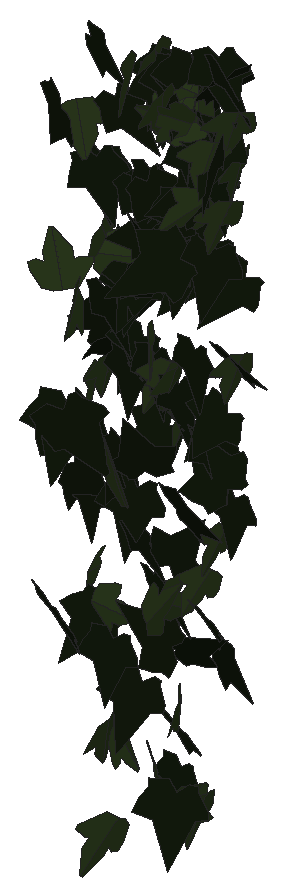
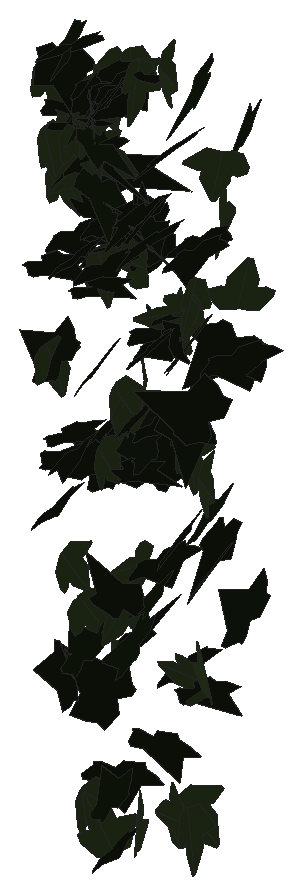
# SketchUp Ruby script. Lengths in inches.
U = 1.inch
M = Sketchup.active_model
def pt(a) = Geom::Point3d.new(a.map { |v| v * U })
def face(e, loops, mat)
  f = e.add_face(loops[0].map { |a| pt(a) })
  loops[1..].each { |l| e.add_face(l.map { |a| pt(a) }).erase! }
  f.material = f.back_material = mat if mat
  f
end
# faces: each face lists its corners as indices into pts; further lists are holes
def faces(e, pts, list, mat = nil) = list.each { |f| face(e, (f[0].is_a?(Array) ? f : [f]).map { |l| l.map { |i| pts[i] } }, mat) }
# xy, xz, yz: faces in a plane at the given z, y or x. An outline is a flat list of corners, or four numbers for a rectangle; further outlines are holes
def ring(l) = l.size == 4 ? [[l[0], l[1]], [l[2], l[1]], [l[2], l[3]], [l[0], l[3]]] : l.each_slice(2).to_a
def flat(e, list, mat, &to3) = list.each { |f| face(e, (f[0].is_a?(Array) ? f : [f]).map { |l| ring(l).map { |u, v| to3.(u, v) } }, mat) }
def xy(e, z, list, mat = nil) = flat(e, list, mat) { |x, y| [x, y, z] }
def xz(e, y, list, mat = nil) = flat(e, list, mat) { |x, z| [x, y, z] }
def yz(e, x, list, mat = nil) = flat(e, list, mat) { |y, z| [x, y, z] }
def lines(e, pts, list) = list.each { |a, b| e.add_line(pt(pts[a]), pt(pts[b])) }
# prism: a flat outline (further loops are holes) pulled along v
def prism(e, loops, v, mat = nil)
  f = face(e, loops, mat); d = Geom::Vector3d.new(v.map { |x| x * U })
  f.pushpull(f.normal.samedirection?(d) ? d.length : -d.length)
end
def box(e, o, s, mat = nil) = prism(e, [[o, [o[0] + s[0], o[1], o[2]], [o[0] + s[0], o[1] + s[1], o[2]], [o[0], o[1] + s[1], o[2]]]], [0, 0, s[2]], mat)
def at(x, y, z, deg = 0) = Geom::Transformation.translation(pt([x, y, z])) * Geom::Transformation.rotation(ORIGIN, Z_AXIS, deg.degrees)
def axes(o, x, y, z) = Geom::Transformation.new([*x, 0, *y, 0, *z, 0, *pt(o).to_a, 1])
def part(name) = M.definitions.add(name)
# library, detail: a bought-in or finely detailed component or shape, given as its bounding box
def library(name, o, s) = part(name).tap { |d| box(d.entities, o, s) }
def detail(e, o, s) = box(e.add_group.entities, o, s)
def put(e, d, t, mat = nil) = e.add_instance(d, t).tap { |i| i.material = mat if mat }
def group(e, t, mat = nil) = e.add_group.tap { |g| g.transformation = t; g.material = mat if mat }.entities
root = M.entities
M.materials.add("efeu1").color = [18, 25, 13]
M.materials.add("efeu2").color = [43, 57, 29]
c1 = part("ivyleaf_10")
p = [[0,0.5,-0.03],[-0.0625,2.02,-0.43],[-0.19,2.01,-0.46],[-0.54,1.05,-0.29],[-0.52,0.625,-0.18],[-0.83,0.76,-0.28],
  [-1.16,0.64,-0.33],[-1.15,0.33,-0.24],[-0.77,-0.39,0.02],[-0.3,-0.51,0.16],[0.04,-0.48,0.23],[-0.02,2.01,-0.4375],
  [-0.06,2.01,-0.43],[0.04,-0.49,0.23],[0.67,-0.49,0.14],[1.38,0.36,-0.2],[1.375,0.51,-0.24],[0.81,0.65,-0.19],
  [0.62,0.59,-0.15],[0.6,1.09,-0.28],[0.5,1.23,-0.31]]
faces(c1.entities,p,[[0,1,2,3,4,5,6,7,8,9,10],[11,12,0,13,14,15,16,17,18,19,20]],"efeu2")
c2 = part("ivyleaf_9")
p = [[1.54,2.16,1.25],[1.36,2.04,1.19],[-0.21,0.99,0.68],[-0.71,1.11,0.82],[-0.85,0.86,0.67],[-0.8,0.17,0.21],
  [-0.9,-0.01,0.1],[-0.67,-0.16,-0.02],[-0.08,-0.08,-0.05],[-0.03,-0.6,-0.4],[0.65,-0.88,-0.66],[0.83,-0.6,-0.49],
  [1.29,-0.42,-0.43],[1.8125,-0.07,-0.26],[1.21,0.44,0.15]]
faces(c2.entities,p,[[0,1,2,3,4,5,6,7,8,9,10,11,12,13,14]],"efeu1")
put(root,c1,axes([528.05,122.93,226.38],[-0.82158,0.69084,-0.51551],[-0.39036,0.33675,1.07342],[0.76852,0.90958,-0.00587]))
put(root,c1,axes([524.125,124.99,233.47],[-0.13432,0.38401,-1.0691],[0.2143,-1.04865,-0.40359],[-1.11557,-0.24768,0.05119]))
put(root,c2,axes([523.31,125.25,227.76],[-0.44076,-1.03489,-0.11415],[0.04301,0.10575,-1.12484],[1.04028,-0.44285,-0.00185]))
put(root,c2,axes([523.81,124.54,228.03],[-0.22106,-0.48104,-1.08794],[0.56667,0.93036,-0.5265],[1.0459,-0.60574,0.05532]))
put(root,c2,axes([521.58,126.45,217.07],[0.38586,-0.75336,0.79815],[0.49333,-0.63671,-0.83948],[0.98042,0.61688,0.10828]))
put(root,c1,axes([524.64,126.52,207.5],[-0.23778,-0.90858,0.68289],[-0.07381,-0.68385,-0.93556],[1.13419,-0.23498,0.08228]))
put(root,c2,axes([527.59,127.25,235.54],[-0.92071,-0.44136,0.53496],[-0.48506,-0.22567,-1.02101],[0.49568,-1.04065,-0.00548]))
put(root,c2,axes([520.4,128.47,239.76],[0.04113,-0.61141,0.89089],[0.11295,-0.88422,-0.61205],[1.07459,0.11634,0.03024]))
put(root,c2,axes([526.9,128.12,209.15],[-0.64224,-0.76315,-0.42743],[0.2906,0.314,-0.99726],[0.82502,-0.70468,0.01853]))
put(root,c2,axes([527,128.16,222.95],[0.48538,-0.48585,0.89186],[0.66554,-0.5945,-0.68607],[0.76716,0.82315,0.03091]))
put(root,c2,axes([523.32,128.32,215.22],[-0.15697,-0.9643,0.02792],[-0.00409,-0.02762,-0.97699],[0.9647,-0.15702,0.0004]))
put(root,c1,axes([527.36,127.64,213.96],[0.4042,-0.81495,-0.41775],[-0.07641,0.42502,-0.90308],[0.91259,0.39654,0.10941]))
put(root,c1,axes([520.98,127.72,232.23],[0.76284,0.74931,0.11152],[-0.08398,-0.07364,1.06928],[0.7529,-0.76742,0.00628]))
put(root,c1,axes([526.41,127.1,218.1],[0.03617,0.22167,-0.982],[0.18316,0.96479,0.22453],[0.98991,-0.18661,-0.00566]))
put(root,c2,axes([525.27,127.54,233.92],[0.06716,0.70227,-0.87889],[-0.07759,0.88125,0.69822],[1.12232,0.0189,0.10086]))
put(root,c1,axes([527.23,129.23,237.1875],[-0.20712,-0.47742,0.89381],[-0.34689,-0.82377,-0.52039],[0.9521,-0.40399,0.00484]))
put(root,c2,axes([525.67,129.17,215.49],[-0.16332,-1.08391,-0.06907],[0.01401,-0.07194,1.09587],[-1.08602,0.16207,0.02452]))
put(root,c1,axes([526.28,129.19,240.88],[-0.45119,-0.04257,-0.89484],[-0.78436,-0.4653,0.41762],[-0.43282,0.88759,0.17601]))
put(root,c2,axes([524.46,129.01,223.66],[0.66107,0.19822,0.71645],[-0.72383,-0.04672,0.6808],[0.16931,-0.97372,0.11318]))
put(root,c1,axes([525.6,128.76,241.8125],[0.01224,-0.98949,-0.23253],[0.04073,0.23284,-0.98866],[1.01563,0.00259,0.04245]))
put(root,c1,axes([523.38,129.43,242.38],[0.36501,-0.60969,0.76872],[0.47856,-0.60538,-0.70737],[0.85653,0.59806,0.06763]))
put(root,c2,axes([524.375,129.59,233.91],[-0.36953,-0.23006,0.96265],[0.47782,-0.94135,-0.04155],[0.86678,0.42084,0.43331]))
put(root,c1,axes([527.19,129.4375,208.32],[0.05239,-1.06977,0.20179],[0.0094,-0.20157,-1.07105],[1.08859,0.05322,-0.00046]))
put(root,c2,axes([521.48,129.8125,215.42],[-0.75245,-0.58306,0.12384],[-0.09953,-0.07374,-0.95191],[0.5877,-0.759,-0.00265]))
put(root,c1,axes([527.54,129.65,239.68],[-0.56199,-0.75208,0.30846],[-0.03648,-0.35129,-0.92297],[0.81206,-0.53626,0.17201]))
put(root,c1,axes([520.67,129.3,239.35],[0.73743,0.69098,0.18934],[0.1294,0.13879,-1.01049],[-0.70467,0.74859,0.01258]))
put(root,c2,axes([526.95,129.5625,237.52],[-0.94111,0.29635,0.29843],[-0.28157,0.09938,-0.98662],[-0.31242,-0.98228,-0.00978]))
put(root,c2,axes([520.66,129.97,221.14],[0.21557,-0.86108,0.23473],[0.02361,-0.23589,-0.88703],[0.89218,0.2143,-0.03324]))
put(root,c2,axes([525.78,130.06,233.94],[-0.22906,-0.94928,0.0558],[0.0273,-0.06394,-0.97565],[0.95053,-0.22693,0.04147]))
put(root,c2,axes([521.81,129.75,230.93],[0.5139,-0.90185,-0.06053],[-0.02558,0.0551,-1.03798],[0.90352,0.51451,0.00505]))
put(root,c2,axes([523.51,129.92,212.54],[-0.86262,-0.51536,-0.33613],[0.28798,0.17335,-1.00485],[0.54373,-0.90942,-0.00106]))
put(root,c2,axes([527.5,129.93,239.87],[-0.6685,0.03235,-0.80034],[0.79361,-0.11444,-0.66751],[-0.10848,-1.03651,0.04872]))
put(root,c1,axes([524.52,129.68,233.44],[0.06923,-0.03854,1.09488],[1.09536,0.02307,-0.06845],[-0.0206,1.09682,0.03991]))
put(root,c1,axes([525.54,129,217.65],[-0.15498,-0.64223,-0.88155],[0.24334,0.8476,-0.66028],[1.06319,-0.28762,0.02262]))
put(root,c1,axes([521.6,129.79,215.79],[-0.06161,-0.14923,-0.94753],[0.91503,-0.29398,-0.0132],[-0.28775,-0.90288,0.16091]))
put(root,c2,axes([522.63,130.26,227.44],[0.11146,-0.86515,0.39633],[0.08959,-0.38773,-0.87156],[0.94738,0.13845,0.03579]))
put(root,c2,axes([520.71,129.15,222.49],[0.27625,-0.36518,-0.96289],[-0.57807,0.77007,-0.4579],[0.85227,0.64068,0.00153]))
put(root,c2,axes([525.0625,130.19,235.4],[-0.62155,-0.40287,-0.62601],[0.66837,0.05712,-0.70038],[0.32782,-0.88031,0.24104]))
put(root,c1,axes([525.47,129.42,240.3125],[0.99684,0.20328,-0.47278],[0.40809,0.31566,0.99617],[0.31354,-1.05715,0.20654]))
put(root,c1,axes([527.91,130.18,236.74],[-0.22239,-0.9539,0.34583],[-0.03989,-0.34555,-0.97876],[1.01387,-0.22283,0.03735]))
put(root,c2,axes([521.3,129.58,242.93],[0.78232,-0.42719,-0.51522],[-0.41356,0.31458,-0.8888],[0.52621,0.88233,0.06745]))
put(root,c2,axes([524.18,129.78,234.72],[-0.74461,0.53945,0.32451],[-0.31965,0.10905,-0.91471],[-0.54234,-0.8049,0.09357]))
put(root,c1,axes([522.03,130.21,209.45],[0.24571,-0.08568,1.02242],[1.00044,-0.21322,-0.2583],[0.22761,1.02969,0.03159]))
put(root,c2,axes([527.11,130.45,234.33],[-0.34737,-0.96548,-0.06332],[0.01068,0.06345,-1.026],[0.96749,-0.34734,-0.01141]))
put(root,c1,axes([526.03,130.28,241.25],[-0.70517,-0.59037,0.36839],[-0.149,-0.38422,-0.90094],[0.67974,-0.69668,0.18469]))
put(root,c2,axes([527.4375,130.51,240.04],[-0.67206,-0.71263,-0.16812],[0.15229,0.08717,-0.97825],[0.71618,-0.68726,0.05026]))
put(root,c1,axes([523.59,130.53,228.95],[-0.30792,0.42784,-0.84012],[0.33795,-0.77497,-0.51853],[-0.88013,-0.44725,0.09482]))
put(root,c1,axes([525.66,130.1,207.25],[-0.77015,-0.42954,0.52529],[0.51386,0.14972,0.87584],[-0.44314,0.92013,0.1027]))
put(root,c2,axes([524.43,130.48,241.76],[-0.20291,-0.97376,-0.16203],[0.02509,0.16028,-0.99465],[0.98683,-0.2043,-0.00803]))
put(root,c1,axes([524.94,130.29,227.68],[0.108,-0.95409,0.09059],[0.01397,-0.08959,-0.96018],[0.95828,0.10883,0.00378]))
put(root,c1,axes([528.32,130.29,241.16],[-0.47391,-0.85715,0.19311],[-0.10186,-0.16433,-0.97939],[0.87271,-0.48464,-0.00945]))
put(root,c2,axes([522.7,130.69,221.24],[-0.30401,-1.01642,-0.05268],[0.01513,0.05047,-1.06091],[1.01767,-0.30439,0.00003]))
put(root,c1,axes([523.87,130.52,208.03],[-0.58296,0.44962,0.68947],[0.55492,-0.40933,0.73613],[0.60794,0.80477,-0.01078]))
put(root,c2,axes([522.93,130.25,219.67],[0.61871,-0.66751,-0.06586],[-0.01633,0.07458,-0.90933],[0.67055,0.61772,0.03862]))
put(root,c1,axes([524.24,130.68,227.51],[-0.24512,-0.73679,0.54659],[0.02961,-0.57182,-0.75753],[0.91692,-0.1785,0.17058]))
put(root,c2,axes([520.11,130.88,223.9],[0.07427,-0.79347,0.61327],[0.17046,-0.59601,-0.79178],[0.98825,0.16243,0.09049]))
put(root,c2,axes([527.8,130.26,223.42],[-0.85081,-0.62406,-0.02234],[-0.00632,-0.02913,1.05495],[-0.62442,0.8506,0.01975]))
put(root,c2,axes([524.23,130.82,224.82],[-0.77445,-0.42705,0.3107],[-0.23226,-0.21986,-0.88113],[0.4743,-0.80496,0.07584]))
put(root,c1,axes([521.46,130.24,209.65],[0.09529,-1.02806,-0.19432],[-0.02142,0.19317,-1.03247],[1.04605,0.09761,-0.00344]))
put(root,c2,axes([525.75,130.8,228.875],[0.22779,-0.91816,0.22903],[0.02551,-0.22953,-0.94553],[0.94595,0.22729,-0.02966]))
put(root,c2,axes([521.65,131.11,222.34],[-0.03199,-0.80115,0.61232],[-0.02216,-0.61192,-0.80178],[1.00811,-0.03887,0.00181]))
put(root,c1,axes([525.78,130.48,233.55],[-0.10448,-0.95509,0.05949],[-0.00492,-0.05931,-0.96079],[0.95693,-0.10458,0.00156]))
put(root,c2,axes([522.03,130.28,240],[0.49496,-0.78164,-0.39133],[0.05385,0.47612,-0.88289],[0.87247,0.41404,0.2765]))
put(root,c1,axes([520.22,130.84,216.39],[0.18752,-0.56593,-0.73593],[0.42453,-0.61542,0.58143],[-0.82561,-0.44498,0.13182]))
put(root,c2,axes([522.86,130.9375,231.7],[-0.49023,-0.83607,0.06848],[-0.01952,-0.06793,-0.96904],[0.83865,-0.49031,0.01748]))
put(root,c2,axes([524.875,130.875,242.01],[-0.33972,-0.94987,-0.04401],[0.01231,0.04234,-1.00879],[0.95081,-0.33994,-0.00267]))
put(root,c1,axes([521.38,130.09,233.51],[0.0962,-0.84611,-0.48465],[0.13742,0.49391,-0.835],[0.96536,0.01401,0.16716]))
put(root,c2,axes([525.125,130.83,235.82],[-0.18444,-0.95277,-0.0685],[0.01328,0.0672,-0.97045],[0.95513,-0.18492,0.00027]))
put(root,c2,axes([524.42,130.95,242.09],[-0.50013,-0.85702,0.03239],[-0.01383,-0.02943,-0.99227],[0.85752,-0.50032,0.00289]))
put(root,c2,axes([523.75,130.28,236.51],[0.40042,-0.75278,-0.57248],[-0.06336,0.59893,-0.83188],[0.94361,0.35966,0.18707]))
put(root,c1,axes([520.18,131,225.7],[0.35334,-0.64675,0.74932],[0.50447,-0.56689,-0.72717],[0.85164,0.60413,0.11985]))
put(root,c2,axes([526.26,130.79,236.04],[-0.96258,-0.14515,0.08264],[-0.08254,-0.00689,-0.97345],[0.14521,-0.9661,-0.00547]))
put(root,c2,axes([525.4375,131.12,242.17],[-0.35754,-1.00167,0.1176],[-0.01994,-0.11773,-1.06337],[1.00835,-0.3575,0.02067]))
put(root,c2,axes([524.83,131.23,241.44],[-0.03387,-0.96377,0.45458],[-0.00158,-0.45476,-0.96428],[1.0656,-0.03131,0.01302]))
put(root,c2,axes([524.86,130.84,226.89],[0.24209,-0.91626,-0.03594],[-0.00899,0.0348,-0.9477],[0.91692,0.24226,0.0002]))
put(root,c2,axes([520.6,130.7,236.4],[0.00852,-0.90825,-0.39058],[0.06651,0.39023,-0.906],[0.98643,-0.01847,0.06446]))
put(root,c2,axes([524.73,131.23,241.17],[-0.33359,-0.91813,0.23362],[-0.01572,-0.24228,-0.97461],[0.94725,-0.32735,0.0661]))
put(root,c1,axes([526.15,131,218.08],[-0.32144,-0.6764,0.52244],[-0.08025,-0.53181,-0.73791],[0.85089,-0.30568,0.12777]))
put(root,c2,axes([522.33,131.09,231.42],[-0.21665,-0.94448,0.04012],[-0.01023,-0.03882,-0.96901],[0.94528,-0.21689,-0.00129]))
put(root,c1,axes([521.67,130.15,232.52],[-0.0094,-0.27296,-1.00474],[0.90248,0.4989,-0.14398],[0.51917,-0.87218,0.23209]))
put(root,c2,axes([522.85,130.83,226.6],[0.73925,-0.58942,0.40228],[0.32494,-0.23766,-0.94534],[0.63535,0.80736,0.01541]))
put(root,c2,axes([526.56,130.99,237.91],[0.21715,-0.97144,-0.05633],[-0.00734,0.05608,-0.9954],[0.97305,0.21721,0.00506]))
put(root,c2,axes([523.4,131.06,227.73],[0.20158,-0.93513,0.04936],[0.00851,-0.04866,-0.95661],[0.93639,0.20175,-0.00194]))
put(root,c2,axes([525.71,131.07,238.65],[-0.06591,-0.99389,-0.09302],[0.01592,0.09216,-0.99603],[0.99811,-0.0671,0.00975]))
put(root,c2,axes([525.63,131.32,232.78],[-0.68562,-0.64324,0.22955],[-0.06176,-0.26554,-0.92855],[0.68018,-0.6725,0.14708]))
put(root,c1,axes([521.11,130.77,226.89],[-0.01628,-0.94355,-0.0167],[0.00042,0.01669,-0.9437],[0.9437,-0.01628,0.00014]))
put(root,c2,axes([527.95,131.28,233.03],[-0.75459,-0.5788,0.19035],[-0.11257,-0.16534,-0.94902],[0.5988,-0.76046,0.06146]))
put(root,c2,axes([523.56,130.96,217.2],[0.67614,-0.75593,0.20134],[0.14787,-0.13782,-1.01404],[0.76818,0.69189,0.01798]))
put(root,c2,axes([527.51,131.27,222.17],[0.02026,-0.9087,0.20747],[0.02489,-0.20692,-0.90871],[0.93175,0.02528,0.01976]))
put(root,c2,axes([526.57,130.99,224.94],[0.17207,-0.9237,-0.18365],[-0.03059,0.18111,-0.93959],[0.94128,0.17475,0.00304]))
put(root,c2,axes([525.84,131.54,240.76],[-0.18054,-0.25589,0.9416],[-0.51829,-0.78618,-0.31303],[0.82672,-0.54875,0.00938]))
put(root,c1,axes([523.83,130.53,242.65],[-0.0242,-0.91499,-0.42909],[0.07728,0.42628,-0.91336],[1.00765,-0.05466,0.05974]))
put(root,c2,axes([523.19,131.11,236.45],[0.31987,-0.93261,0.02621],[0.00801,-0.02496,-0.98594],[0.93294,0.31997,-0.00052]))
put(root,c2,axes([524.59,130.68,218.44],[-0.44338,0.12379,0.79146],[0.73261,-0.30329,0.45785],[0.32407,0.855,0.04782]))
put(root,c2,axes([525.96,131.34,215.92],[0.05094,-0.55307,0.74732],[0.45961,-0.63561,-0.50172],[0.80816,0.39634,0.23823]))
put(root,c2,axes([522.49,130.4,230.99],[0.31348,0.13519,0.89793],[-0.53647,0.794,0.06774],[-0.73264,-0.52356,0.3346]))
put(root,c2,axes([526.94,131.04,242.9],[0.63079,-0.76719,0.12365],[0.08018,-0.09415,-0.99322],[0.77295,0.63587,0.00212]))
put(root,c2,axes([527.02,131.02,214.77],[0.12021,-0.04949,-0.95752],[0.94578,0.16459,0.11023],[0.15745,-0.9509,0.06891]))
put(root,c2,axes([526.79,131.12,243.17],[0.02427,-0.9734,-0.24861],[0.20263,0.24831,-0.95246],[0.984,-0.02713,0.20227]))
put(root,c2,axes([524.875,130.8,214.3125],[0.84759,0.43122,-0.43161],[0.38137,0.20222,0.95095],[0.47623,-0.92941,0.00665]))
put(root,c2,axes([527.32,131.2,228.8],[0.34849,-0.52864,0.7423],[0.61272,-0.45235,-0.60981],[0.67457,0.68398,0.17042]))
put(root,c1,axes([526.625,130.36,238],[-0.23957,-0.56106,-0.84043],[0.41317,0.73384,-0.60768],[0.92217,-0.47455,0.05393]))
put(root,c1,axes([527.76,131.19,228.9],[-0.15203,-0.90138,0.25363],[0.01771,-0.25967,-0.91224],[0.93622,-0.14146,0.05844]))
put(root,c2,axes([526.03,131.45,240.12],[0.34484,-0.79158,0.49115],[0.1816,-0.45655,-0.86333],[0.9137,0.38949,-0.01378]))
put(root,c1,axes([525.85,130.96,241.23],[0.47392,-0.88313,-0.08799],[0.08229,0.14305,-0.99249],[0.88368,0.46031,0.13961]))
put(root,c2,axes([526.71,131.6,225.92],[-0.58251,-0.67175,0.29183],[-0.09144,-0.30325,-0.88057],[0.72667,-0.57664,0.12313]))
put(root,c2,axes([522.59,130.89,236.01],[0.3945,-0.79386,-0.42932],[0.07053,0.49423,-0.84907],[0.89975,0.30933,0.2548]))
put(root,c2,axes([524.96,131.37,234.03],[-0.17738,-0.95115,-0.13532],[0.02971,0.13211,-0.96754],[0.96027,-0.17979,0.00494]))
put(root,c2,axes([524.43,131.52,209.93],[0.0113,-0.55256,0.69409],[0.40567,-0.61411,-0.49549],[0.78899,0.32366,0.24482]))
put(root,c2,axes([526.33,131.58,233.93],[-0.10281,-0.91811,0.24993],[0.06847,-0.25787,-0.91911],[0.94905,-0.08085,0.09339]))
put(root,c2,axes([520.45,131.28,236.16],[-0.04808,-0.95101,-0.24874],[0.02095,0.24799,-0.95219],[0.98278,-0.05181,0.00812]))
put(root,c2,axes([526.37,131.64,240.03],[-0.68351,-0.71274,-0.00371],[0.18044,-0.16807,-0.95624],[0.68953,-0.66254,0.24656]))
put(root,c2,axes([522.21,131.66,227.95],[-0.30332,-0.84907,0.25897],[-0.05213,-0.25616,-0.90092],[0.88616,-0.30569,0.03564]))
put(root,c1,axes([526.29,131.36,239.48],[-0.26183,-0.87203,0.36129],[-0.03961,-0.36445,-0.90837],[0.94308,-0.25741,0.06216]))
put(root,c2,axes([525.72,130.48,236.99],[-0.09714,0.9131,0.32755],[-0.22391,0.29919,-0.90045],[-0.94387,-0.16495,0.1799]))
put(root,c1,axes([526.61,131.51,220.13],[0.01683,-0.76707,0.51228],[0.10011,-0.50782,-0.76369],[0.91696,0.06952,0.07397]))
put(root,c1,axes([525.875,130.78,240.54],[-0.20449,-0.87716,-0.45135],[0.11811,0.43586,-0.90057],[0.97937,-0.23571,0.01436]))
put(root,c2,axes([525.67,131.42,239.79],[-0.77423,0.41184,-0.4684],[0.2639,-0.46021,-0.84084],[-0.56513,-0.77913,0.24907]))
put(root,c2,axes([527.3,130.9375,242.4375],[-0.07855,0.92193,-0.35814],[0.01358,-0.35823,-0.92513],[-0.98895,-0.07814,0.01575]))
put(root,c1,axes([524.73,131.61,225.57],[0.10897,-0.7675,0.5544],[0.24665,-0.51578,-0.76252],[0.91411,0.23066,0.13966]))
put(root,c1,axes([527.82,131.25,238.63],[0.17516,-0.98673,0.0136],[0.00223,-0.01342,-1.00216],[0.98682,0.17518,-0.00015]))
put(root,c2,axes([524.28,131.64,207.99],[0.0082,-0.84083,0.22261],[-0.01136,-0.22271,-0.84077],[0.86972,0.00502,-0.01308]))
put(root,c2,axes([521.18,130.65,228.08],[0.07058,0.94602,0.02335],[-0.00446,0.02374,-0.94863],[-0.9463,0.07045,0.00622]))
put(root,c2,axes([522.39,131.83,231.25],[-0.20771,-0.83885,0.42478],[0.02831,-0.44041,-0.85586],[0.93985,-0.17212,0.11966]))
put(root,c2,axes([520.41,130.65,228.28],[0.14871,-0.0125,1.04738],[1.01384,0.26756,-0.14076],[-0.26322,1.02349,0.04959]))
